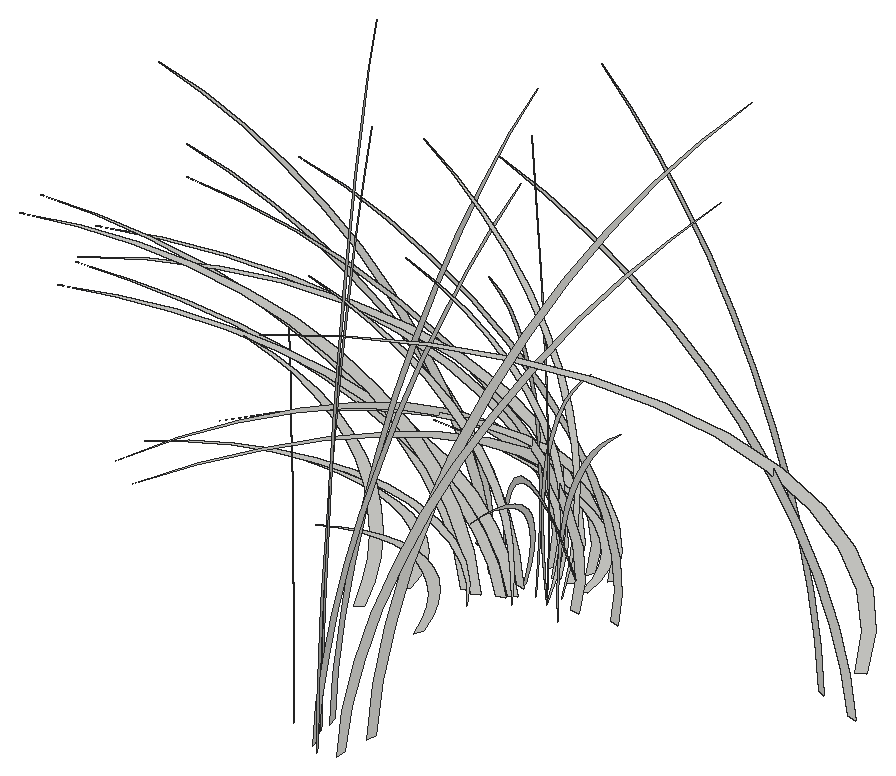
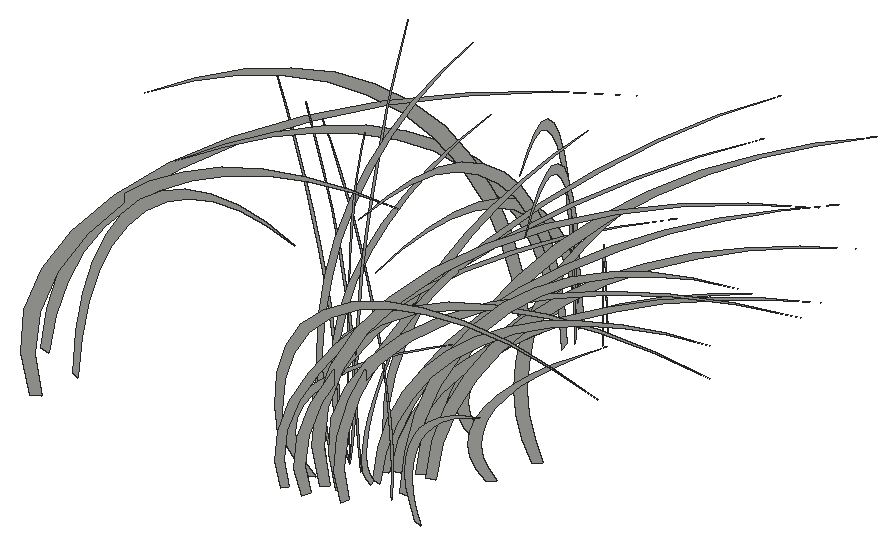
# SketchUp Ruby script. Lengths in inches.
U = 1.inch
M = Sketchup.active_model
def pt(a) = Geom::Point3d.new(a.map { |v| v * U })
def face(e, loops, mat)
  f = e.add_face(loops[0].map { |a| pt(a) })
  loops[1..].each { |l| e.add_face(l.map { |a| pt(a) }).erase! }
  f.material = f.back_material = mat if mat
  f
end
# faces: each face lists its corners as indices into pts; further lists are holes
def faces(e, pts, list, mat = nil) = list.each { |f| face(e, (f[0].is_a?(Array) ? f : [f]).map { |l| l.map { |i| pts[i] } }, mat) }
# xy, xz, yz: faces in a plane at the given z, y or x. An outline is a flat list of corners, or four numbers for a rectangle; further outlines are holes
def ring(l) = l.size == 4 ? [[l[0], l[1]], [l[2], l[1]], [l[2], l[3]], [l[0], l[3]]] : l.each_slice(2).to_a
def flat(e, list, mat, &to3) = list.each { |f| face(e, (f[0].is_a?(Array) ? f : [f]).map { |l| ring(l).map { |u, v| to3.(u, v) } }, mat) }
def xy(e, z, list, mat = nil) = flat(e, list, mat) { |x, y| [x, y, z] }
def xz(e, y, list, mat = nil) = flat(e, list, mat) { |x, z| [x, y, z] }
def yz(e, x, list, mat = nil) = flat(e, list, mat) { |y, z| [x, y, z] }
def lines(e, pts, list) = list.each { |a, b| e.add_line(pt(pts[a]), pt(pts[b])) }
# prism: a flat outline (further loops are holes) pulled along v
def prism(e, loops, v, mat = nil)
  f = face(e, loops, mat); d = Geom::Vector3d.new(v.map { |x| x * U })
  f.pushpull(f.normal.samedirection?(d) ? d.length : -d.length)
end
def box(e, o, s, mat = nil) = prism(e, [[o, [o[0] + s[0], o[1], o[2]], [o[0] + s[0], o[1] + s[1], o[2]], [o[0], o[1] + s[1], o[2]]]], [0, 0, s[2]], mat)
def at(x, y, z, deg = 0) = Geom::Transformation.translation(pt([x, y, z])) * Geom::Transformation.rotation(ORIGIN, Z_AXIS, deg.degrees)
def axes(o, x, y, z) = Geom::Transformation.new([*x, 0, *y, 0, *z, 0, *pt(o).to_a, 1])
def part(name) = M.definitions.add(name)
# library, detail: a bought-in or finely detailed component or shape, given as its bounding box
def library(name, o, s) = part(name).tap { |d| box(d.entities, o, s) }
def detail(e, o, s) = box(e.add_group.entities, o, s)
def put(e, d, t, mat = nil) = e.add_instance(d, t).tap { |i| i.material = mat if mat }
def group(e, t, mat = nil) = e.add_group.tap { |g| g.transformation = t; g.material = mat if mat }.entities
root = M.entities
g1 = group(root,at(15.17,758.32,-58.625))
p = [[-6.5,7.92,6.04],[-5.63,6.85,6],[-4.77,5.81,5.85],[-3.94,4.8,5.6],[-3.16,3.84,5.25],[-2.4375,2.97,4.81],
  [-1.79,2.18,4.28],[-1.23,1.5,3.68],[-0.77,0.9375,3.02],[-0.42,0.51,2.3],[-0.18,0.22,1.55],[-0.06,0.07,0.78],
  [-0.06,0.07,0],[0,0,0.8],[-0.08,0.09,1.59],[-0.28,0.35,2.36],[-0.62,0.76,3.1],[-1.08,1.3125,3.79],
  [-1.64,2,4.41],[-2.31,2.81,4.94],[-3.05,3.72,5.38],[-3.86,4.7,5.72],[-4.72,5.75,5.94],[-5.61,6.83,6.05]]
faces(g1,p,[[0,1,2,3,4,5,6,7,8,9,10,11,12,13,14,15,16,17,18,19,20,21,22,23]])
g2 = group(root,at(15.29,769.34,-58.625))
p = [[-0.14,-0.48,0],[-0.0625,-0.21,0],[0,0,1.01],[-0.03,-0.09,2.03],[-0.14,-0.47,3.02],[-0.33,-1.14,3.98],
  [-0.61,-2.08,4.86],[-0.95,-3.26,5.65],[-1.37,-4.67,6.34],[-1.83,-6.26,6.89],[-2.34,-7.99,7.31],[-2.87,-9.82,7.58],
  [-3.42,-11.7,7.68],[-3.98,-13.6,7.63],[-3.43,-11.74,7.64],[-2.89,-9.9,7.5],[-2.375,-8.12,7.21],[-1.88,-6.44,6.78],
  [-1.43,-4.91,6.22],[-1.04,-3.55,5.54],[-0.7,-2.39,4.76],[-0.43,-1.48,3.89],[-0.24,-0.8125,2.96],[-0.125,-0.42,1.99],
  [-0.09,-0.31,0.99]]
faces(g2,p,[[0,1,2,3,4,5,6,7,8,9,10,11,12,13,14,15,16,17,18,19,20,21,22,23,24]])
g3 = group(root,at(16.34,769.67,-58.625))
p = [[-0.18,-0.47,0],[-0.08,-0.21,0],[0,0,0.88],[-0.03,-0.08,1.76],[-0.17,-0.46,2.63],[-0.42,-1.11,3.46],
  [-0.77,-2.02,4.23],[-1.2,-3.18,4.92],[-1.72,-4.55,5.51],[-2.3,-6.1,6],[-2.94,-7.78,6.36],[-3.62,-9.57,6.59],
  [-4.31,-11.41,6.6875],[-5.01,-13.25,6.64],[-4.32,-11.44,6.65],[-3.65,-9.65,6.53],[-2.99,-7.91,6.28],[-2.37,-6.28,5.9],
  [-1.81,-4.78,5.41],[-1.31,-3.46,4.82],[-0.88,-2.33,4.14],[-0.54,-1.4375,3.39],[-0.3,-0.79,2.58],[-0.16,-0.41,1.73],
  [-0.11,-0.3,0.86]]
faces(g3,p,[[0,1,2,3,4,5,6,7,8,9,10,11,12,13,14,15,16,17,18,19,20,21,22,23,24]])
g4 = group(root,at(14.92,764.6875,-58.625))
p = [[-1.5,-3.28,3.96],[-1.23,-2.68,3.71],[-0.98,-2.14,3.43],[-0.76,-1.66,3.13],[-0.57,-1.25,2.82],[-0.42,-0.91,2.49],
  [-0.29,-0.64,2.15],[-0.21,-0.45,1.79],[-0.16,-0.34,1.43],[-0.14,-0.31,1.07],[-0.16,-0.35,0.71],[-0.22,-0.48,0.35],
  [-0.3125,-0.6875,0],[-0.19,-0.42,0],[-0.09,-0.19,0.36],[-0.02,-0.05,0.72],[0,0,1.09],[-0.02,-0.04,1.46],
  [-0.07,-0.16,1.82],[-0.17,-0.37,2.18],[-0.31,-0.67,2.53],[-0.48,-1.05,2.86],[-0.6875,-1.5,3.17],[-0.93,-2.03,3.46],
  [-1.2,-2.62,3.72]]
faces(g4,p,[[0,1,2,3,4,5,6,7,8,9,10,11,12,13,14,15,16,17,18,19,20,21,22,23,24]])
g5 = group(root,at(14.8,766.07,-58.625))
p = [[-6.52,-5.35,4.97],[-5.64,-4.63,4.9375],[-4.78,-3.92,4.82],[-3.95,-3.24,4.61],[-3.16,-2.6,4.32],[-2.44,-2,3.96],
  [-1.79,-1.47,3.52],[-1.23,-1.01,3.03],[-0.77,-0.64,2.48],[-0.42,-0.34,1.9],[-0.18,-0.15,1.28],[-0.06,-0.05,0.64],
  [-0.06,-0.05,0],[0,0,0.65],[-0.08,-0.0625,1.31],[-0.29,-0.23,1.95],[-0.62,-0.51,2.55],[-1.08,-0.89,3.12],
  [-1.65,-1.35,3.625],[-2.3125,-1.9,4.07],[-3.06,-2.51,4.43],[-3.87,-3.18,4.7],[-4.73,-3.89,4.89],[-5.62,-4.62,4.98]]
faces(g5,p,[[0,1,2,3,4,5,6,7,8,9,10,11,12,13,14,15,16,17,18,19,20,21,22,23]])
g6 = group(root,at(14.67,766.7,-58.625))
p = [[-8.75,-5.68,10.42],[-10.07,-6.54,10.69],[-8.79,-5.71,10.36],[-7.56,-4.91,9.9],[-6.38,-4.14,9.32],[-5.27,-3.42,8.62],
  [-4.25,-2.76,7.81],[-3.32,-2.16,6.9],[-2.5,-1.62,5.9],[-1.79,-1.16,4.83],[-1.2,-0.78,3.6875],[-0.74,-0.48,2.49],
  [-0.42,-0.27,1.26],[-0.23,-0.15,0],[0,0,0],[-0.15,-0.1,1.29],[-0.46,-0.3,2.55],[-0.91,-0.59,3.78],
  [-1.5,-0.97,4.95],[-2.23,-1.45,6.04],[-3.07,-2,7.05],[-4.03,-2.62,7.96],[-5.1,-3.31,8.76],[-6.25,-4.06,9.45],
  [-7.47,-4.85,10]]
faces(g6,p,[[0,1,2,3,4,5,6,7,8,9,10,11,12,13,14,15,16,17,18,19,20,21,22,23,24]])
g7 = group(root,at(13.05,764.64,-58.625))
p = [[-2.79,-2.29,8.05],[-2.28,-1.87,7.53],[-1.82,-1.49,6.97],[-1.41,-1.16,6.37],[-1.06,-0.87,5.73],[-0.77,-0.63,5.06],
  [-0.54,-0.45,4.36],[-0.38,-0.32,3.64],[-0.29,-0.24,2.91],[-0.26,-0.21,2.18],[-0.3,-0.25,1.44],[-0.41,-0.34,0.71],
  [-0.58,-0.48,0],[-0.36,-0.29,0],[-0.16,-0.14,0.72],[-0.04,-0.04,1.46],[0,0,2.21],[-0.03,-0.03,2.96],
  [-0.14,-0.11,3.71],[-0.32,-0.26,4.43],[-0.57,-0.47,5.14],[-0.89,-0.73,5.81],[-1.28,-1.05,6.44],[-1.72,-1.42,7.03],
  [-2.23,-1.83,7.57]]
faces(g7,p,[[0,1,2,3,4,5,6,7,8,9,10,11,12,13,14,15,16,17,18,19,20,21,22,23,24]])
g8 = group(root,at(13.05,764.64,-58.625))
p = [[-2.79,-2.29,8.05],[-2.28,-1.87,7.53],[-1.82,-1.49,6.97],[-1.41,-1.16,6.37],[-1.06,-0.87,5.73],[-0.77,-0.63,5.06],
  [-0.54,-0.45,4.36],[-0.38,-0.32,3.64],[-0.29,-0.24,2.91],[-0.26,-0.21,2.18],[-0.3,-0.25,1.44],[-0.41,-0.34,0.71],
  [-0.58,-0.48,0],[-0.36,-0.29,0],[-0.16,-0.14,0.72],[-0.04,-0.04,1.46],[0,0,2.21],[-0.03,-0.03,2.96],
  [-0.14,-0.11,3.71],[-0.32,-0.26,4.43],[-0.57,-0.47,5.14],[-0.89,-0.73,5.81],[-1.28,-1.05,6.44],[-1.72,-1.42,7.03],
  [-2.23,-1.83,7.57]]
faces(g8,p,[[0,1,2,3,4,5,6,7,8,9,10,11,12,13,14,15,16,17,18,19,20,21,22,23,24]])
g9 = group(root,at(16.57,757.49,-58.625))
p = [[-6.9,10.63,10.21],[-7.94,12.23,10.48],[-6.9375,10.68,10.15],[-5.96,9.18,9.7],[-5.03,7.75,9.13],[-4.16,6.41,8.44],
  [-3.35,5.16,7.65],[-2.62,4.03,6.76],[-1.97,3.03,5.78],[-1.41,2.17,4.73],[-0.95,1.46,3.61],[-0.58,0.9,2.44],
  [-0.33,0.5,1.23],[-0.18,0.28,0],[0,0,0],[-0.12,0.1875,1.26],[-0.36,0.56,2.5],[-0.72,1.1,3.7],
  [-1.18,1.82,4.85],[-1.76,2.7,5.92],[-2.43,3.73,6.91],[-3.18,4.9,7.8],[-4.02,6.19,8.59],[-4.93,7.59,9.26],
  [-5.89,9.08,9.8]]
faces(g9,p,[[0,1,2,3,4,5,6,7,8,9,10,11,12,13,14,15,16,17,18,19,20,21,22,23,24]])
g10 = group(root,at(15.48,767.23,-58.625))
p = [[-8.75,-5.68,8.4],[-10.07,-6.54,8.62],[-8.79,-5.71,8.35],[-7.56,-4.91,7.98],[-6.38,-4.14,7.51],[-5.27,-3.42,6.95],
  [-4.25,-2.76,6.3],[-3.32,-2.16,5.5625],[-2.5,-1.62,4.76],[-1.79,-1.16,3.89],[-1.2,-0.78,2.97],[-0.74,-0.48,2.01],
  [-0.42,-0.27,1.02],[-0.23,-0.15,0],[0,0,0],[-0.15,-0.1,1.04],[-0.46,-0.3,2.06],[-0.91,-0.59,3.05],
  [-1.5,-0.97,3.99],[-2.23,-1.45,4.87],[-3.07,-2,5.6875],[-4.03,-2.62,6.42],[-5.1,-3.31,7.07],[-6.25,-4.06,7.62],
  [-7.47,-4.85,8.0625]]
faces(g10,p,[[0,1,2,3,4,5,6,7,8,9,10,11,12,13,14,15,16,17,18,19,20,21,22,23,24]])
g11 = group(root,at(15.93,758.48,-58.625))
p = [[-6.9,10.63,12.66],[-7.94,12.23,12.99],[-6.9375,10.68,12.59],[-5.96,9.18,12.03],[-5.03,7.75,11.32],[-4.16,6.41,10.47],
  [-3.35,5.16,9.49],[-2.62,4.03,8.38],[-1.97,3.03,7.17],[-1.41,2.17,5.87],[-0.95,1.46,4.48],[-0.58,0.9,3.03],
  [-0.33,0.5,1.53],[-0.18,0.28,0],[0,0,0],[-0.12,0.1875,1.57],[-0.36,0.56,3.1],[-0.72,1.1,4.59],
  [-1.18,1.82,6.01],[-1.76,2.7,7.34],[-2.43,3.73,8.57],[-3.18,4.9,9.68],[-4.02,6.19,10.65],[-4.93,7.59,11.48],
  [-5.89,9.08,12.15]]
faces(g11,p,[[0,1,2,3,4,5,6,7,8,9,10,11,12,13,14,15,16,17,18,19,20,21,22,23,24]])
g12 = group(root,at(14.18,768.25,-58.625))
p = [[0.29,-0.25,0],[0.13,-0.11,0],[0,0,0.73],[0.05,-0.05,1.47],[0.28,-0.25,2.2],[0.68,-0.6,2.89],
  [1.24,-1.09,3.53],[1.95,-1.71,4.11],[2.79,-2.45,4.6],[3.74,-3.29,5.01],[4.77,-4.19,5.3125],[5.87,-5.16,5.51],
  [7,-6.15,5.58],[8.13,-7.14,5.55],[7.02,-6.17,5.55],[5.92,-5.2,5.45],[4.85,-4.26,5.24],[3.85,-3.38,4.93],
  [2.93,-2.58,4.52],[2.12,-1.86,4.03],[1.43,-1.26,3.46],[0.88,-0.78,2.83],[0.49,-0.43,2.15],[0.25,-0.22,1.44],
  [0.18,-0.16,0.72]]
faces(g12,p,[[0,1,2,3,4,5,6,7,8,9,10,11,12,13,14,15,16,17,18,19,20,21,22,23,24]])
g13 = group(root,at(14.18,768.25,-58.625))
p = [[0.29,-0.25,0],[0.13,-0.11,0],[0,0,0.73],[0.05,-0.05,1.47],[0.28,-0.25,2.2],[0.68,-0.6,2.89],
  [1.24,-1.09,3.53],[1.95,-1.71,4.11],[2.79,-2.45,4.6],[3.74,-3.29,5.01],[4.77,-4.19,5.3125],[5.87,-5.16,5.51],
  [7,-6.15,5.58],[8.13,-7.14,5.55],[7.02,-6.17,5.55],[5.92,-5.2,5.45],[4.85,-4.26,5.24],[3.85,-3.38,4.93],
  [2.93,-2.58,4.52],[2.12,-1.86,4.03],[1.43,-1.26,3.46],[0.88,-0.78,2.83],[0.49,-0.43,2.15],[0.25,-0.22,1.44],
  [0.18,-0.16,0.72]]
faces(g13,p,[[0,1,2,3,4,5,6,7,8,9,10,11,12,13,14,15,16,17,18,19,20,21,22,23,24]])
g14 = group(root,at(16.26,757.74,-58.625))
p = [[-3.71,12.12,8.88],[-4.26,13.95,9.11],[-3.72,12.18,8.83],[-3.2,10.47,8.4375],[-2.7,8.84,7.94],[-2.23,7.3,7.34],
  [-1.8,5.89,6.66],[-1.41,4.6,5.88],[-1.06,3.46,5.03],[-0.76,2.48,4.12],[-0.51,1.66,3.14],[-0.3125,1.03,2.125],
  [-0.18,0.58,1.07],[-0.1,0.32,0],[0,0,0],[-0.07,0.21,1.1],[-0.19,0.64,2.18],[-0.39,1.26,3.22],
  [-0.64,2.08,4.22],[-0.94,3.08,5.15],[-1.3,4.26,6.01],[-1.71,5.59,6.79],[-2.16,7.0625,7.47],[-2.65,8.65,8.05],
  [-3.16,10.35,8.52]]
faces(g14,p,[[0,1,2,3,4,5,6,7,8,9,10,11,12,13,14,15,16,17,18,19,20,21,22,23,24]])
g15 = group(root,at(14.35,766.6875,-58.625))
p = [[-9.98,-3.05,9.0625],[-11.48,-3.51,9.3],[-10.02,-3.0625,9.01],[-8.61,-2.63,8.61],[-7.27,-2.22,8.1],[-6.01,-1.84,7.5],
  [-4.84,-1.48,6.79],[-3.79,-1.16,6],[-2.85,-0.87,5.14],[-2.04,-0.62,4.2],[-1.37,-0.42,3.21],[-0.84,-0.26,2.17],
  [-0.47,-0.14,1.1],[-0.26,-0.08,0],[0,0,0],[-0.18,-0.05,1.12],[-0.52,-0.16,2.22],[-1.04,-0.32,3.29],
  [-1.71,-0.52,4.3],[-2.54,-0.78,5.26],[-3.5,-1.07,6.13],[-4.6,-1.41,6.93],[-5.8125,-1.78,7.625],[-7.12,-2.18,8.22],
  [-8.52,-2.6,8.7]]
faces(g15,p,[[0,1,2,3,4,5,6,7,8,9,10,11,12,13,14,15,16,17,18,19,20,21,22,23,24]])
g16 = group(root,at(17.09,757.67,-58.625))
p = [[0.99,12.64,10.21],[1.14,14.54,10.48],[1,12.7,10.15],[0.86,10.91,9.7],[0.72,9.21,9.13],[0.6,7.61,8.44],
  [0.48,6.14,7.65],[0.38,4.79,6.76],[0.28,3.61,5.78],[0.2,2.58,4.73],[0.14,1.73,3.61],[0.08,1.07,2.44],
  [0.05,0.6,1.23],[0.03,0.33,0],[0,0,0],[0.02,0.22,1.26],[0.05,0.66,2.5],[0.1,1.3125,3.7],
  [0.17,2.17,4.85],[0.25,3.21,5.92],[0.35,4.4375,6.91],[0.46,5.83,7.8],[0.58,7.36,8.59],[0.71,9.02,9.26],
  [0.85,10.79,9.8]]
faces(g16,p,[[0,1,2,3,4,5,6,7,8,9,10,11,12,13,14,15,16,17,18,19,20,21,22,23,24]])
g17 = group(root,at(13.37,766.15,-58.625))
p = [[-2.79,-2.29,3.96],[-2.28,-1.87,3.71],[-1.82,-1.49,3.43],[-1.41,-1.16,3.13],[-1.06,-0.87,2.82],[-0.77,-0.63,2.49],
  [-0.54,-0.45,2.15],[-0.38,-0.32,1.79],[-0.29,-0.24,1.43],[-0.26,-0.21,1.07],[-0.3,-0.25,0.71],[-0.41,-0.34,0.35],
  [-0.58,-0.48,0],[-0.36,-0.29,0],[-0.16,-0.14,0.36],[-0.04,-0.04,0.72],[0,0,1.09],[-0.03,-0.03,1.46],
  [-0.14,-0.11,1.82],[-0.32,-0.26,2.18],[-0.57,-0.47,2.53],[-0.89,-0.73,2.86],[-1.28,-1.05,3.17],[-1.72,-1.42,3.46],
  [-2.23,-1.83,3.72]]
faces(g17,p,[[0,1,2,3,4,5,6,7,8,9,10,11,12,13,14,15,16,17,18,19,20,21,22,23,24]])
g18 = group(root,at(15.69,766.8,-58.625))
p = [[-4.12,-3.38,9.85],[-3.46,-2.84,9.12],[-2.86,-2.35,8.37],[-2.3125,-1.9,7.59],[-1.82,-1.49,6.8],[-1.39,-1.14,5.99],
  [-1.01,-0.83,5.16],[-0.7,-0.57,4.32],[-0.44,-0.36,3.47],[-0.25,-0.21,2.61],[-0.12,-0.1,1.74],[-0.06,-0.05,0.87],
  [-0.05,-0.04,0],[0,0,0.875],[-0.02,-0.02,1.75],[-0.11,-0.09,2.625],[-0.28,-0.23,3.49],[-0.52,-0.43,4.35],
  [-0.83,-0.68,5.2],[-1.21,-1,6.03],[-1.66,-1.37,6.84],[-2.18,-1.79,7.63],[-2.77,-2.27,8.4],[-3.41,-2.8,9.14]]
faces(g18,p,[[0,1,2,3,4,5,6,7,8,9,10,11,12,13,14,15,16,17,18,19,20,21,22,23]])
g19 = group(root,at(15.69,766.8,-58.625))
p = [[-4.12,-3.38,9.85],[-3.46,-2.84,9.12],[-2.86,-2.35,8.37],[-2.3125,-1.9,7.59],[-1.82,-1.49,6.8],[-1.39,-1.14,5.99],
  [-1.01,-0.83,5.16],[-0.7,-0.57,4.32],[-0.44,-0.36,3.47],[-0.25,-0.21,2.61],[-0.12,-0.1,1.74],[-0.06,-0.05,0.87],
  [-0.05,-0.04,0],[0,0,0.875],[-0.02,-0.02,1.75],[-0.11,-0.09,2.625],[-0.28,-0.23,3.49],[-0.52,-0.43,4.35],
  [-0.83,-0.68,5.2],[-1.21,-1,6.03],[-1.66,-1.37,6.84],[-2.18,-1.79,7.63],[-2.77,-2.27,8.4],[-3.41,-2.8,9.14]]
faces(g19,p,[[0,1,2,3,4,5,6,7,8,9,10,11,12,13,14,15,16,17,18,19,20,21,22,23]])
g20 = group(root,at(17.04,769.59,-58.625))
p = [[-0.22,-0.31,0],[-0.1,-0.14,0],[0,0,0.84],[-0.04,-0.06,1.69],[-0.22,-0.3,2.53],[-0.53,-0.74,3.32],
  [-0.96,-1.34,4.06],[-1.52,-2.11,4.72],[-2.17,-3.02,5.29],[-2.9,-4.04,5.76],[-3.71,-5.16,6.11],[-4.56,-6.34,6.33],
  [-5.43,-7.5625,6.42],[-6.31,-8.79,6.375],[-5.45,-7.59,6.38],[-4.6,-6.4,6.27],[-3.77,-5.25,6.02],[-2.99,-4.16,5.67],
  [-2.28,-3.17,5.2],[-1.65,-2.29,4.63],[-1.11,-1.55,3.98],[-0.6875,-0.95,3.25],[-0.38,-0.53,2.47],[-0.2,-0.27,1.66],
  [-0.14,-0.2,0.83]]
faces(g20,p,[[0,1,2,3,4,5,6,7,8,9,10,11,12,13,14,15,16,17,18,19,20,21,22,23,24]])
g21 = group(root,at(15.28,766.97,-58.625))
p = [[-9.98,-3.05,7.31],[-11.48,-3.51,7.5],[-10.02,-3.0625,7.27],[-8.61,-2.63,6.94],[-7.27,-2.22,6.54],[-6.01,-1.84,6.04],
  [-4.84,-1.48,5.48],[-3.79,-1.16,4.84],[-2.85,-0.87,4.14],[-2.04,-0.62,3.39],[-1.37,-0.42,2.59],[-0.84,-0.26,1.75],
  [-0.47,-0.14,0.88],[-0.26,-0.08,0],[0,0,0],[-0.18,-0.05,0.9],[-0.52,-0.16,1.79],[-1.04,-0.32,2.65],
  [-1.71,-0.52,3.47],[-2.54,-0.78,4.24],[-3.5,-1.07,4.95],[-4.6,-1.41,5.59],[-5.8125,-1.78,6.15],[-7.12,-2.18,6.63],
  [-8.52,-2.6,7.02]]
faces(g21,p,[[0,1,2,3,4,5,6,7,8,9,10,11,12,13,14,15,16,17,18,19,20,21,22,23,24]])
g22 = group(root,at(25.3,769.83,-58.625))
p = [[-0.46,-0.32,0],[-0.21,-0.14,0],[0,0,1.26],[-0.08,-0.06,2.52],[-0.45,-0.32,3.76],[-1.1,-0.77,4.94],
  [-2.01,-1.4,6.04],[-3.16,-2.2,7.03],[-4.51,-3.15,7.88],[-6.05,-4.22,8.57],[-7.72,-5.39,9.09],[-9.49,-6.625,9.42],
  [-11.32,-7.9,9.56],[-13.15,-9.17,9.49],[-11.35,-7.92,9.51],[-9.57,-6.68,9.33],[-7.85,-5.48,8.97],[-6.23,-4.35,8.44],
  [-4.75,-3.31,7.74],[-3.43,-2.39,6.89],[-2.32,-1.62,5.92],[-1.43,-1,4.84],[-0.79,-0.55,3.68],[-0.41,-0.28,2.47],
  [-0.3,-0.21,1.23]]
faces(g22,p,[[0,1,2,3,4,5,6,7,8,9,10,11,12,13,14,15,16,17,18,19,20,21,22,23,24]])
g23 = group(root,at(16.39,768.85,-58.625))
p = [[-0.39,-0.25,0],[-0.17,-0.11,0],[0,0,1.1875],[-0.07,-0.05,2.38],[-0.38,-0.25,3.56],[-0.93,-0.6,4.68],
  [-1.69,-1.1,5.72],[-2.66,-1.73,6.65],[-3.8,-2.47,7.45],[-5.09,-3.31,8.11],[-6.5,-4.22,8.6],[-7.99,-5.1875,8.91],
  [-9.53,-6.1875,9.04],[-11.07,-7.1875,8.98],[-9.55,-6.2,8.99],[-8.06,-5.23,8.83],[-6.61,-4.29,8.49],[-5.24,-3.41,7.98],
  [-3.99,-2.59,7.32],[-2.89,-1.875,6.52],[-1.95,-1.27,5.6],[-1.2,-0.78,4.58],[-0.66,-0.43,3.48],[-0.34,-0.22,2.34],
  [-0.25,-0.16,1.17]]
faces(g23,p,[[0,1,2,3,4,5,6,7,8,9,10,11,12,13,14,15,16,17,18,19,20,21,22,23,24]])
g24 = group(root,at(17.07,766.87,-58.625))
p = [[4.46,-2.93,8.37],[3.74,-2.46,7.75],[3.09,-2.03,7.11],[2.5,-1.64,6.45],[1.97,-1.29,5.78],[1.5,-0.98,5.09],
  [1.09,-0.72,4.39],[0.75,-0.49,3.67],[0.48,-0.31,2.95],[0.27,-0.18,2.22],[0.13,-0.09,1.48],[0.0625,-0.04,0.74],
  [0.06,-0.04,0],[0,0,0.74],[0.02,-0.01,1.49],[0.12,-0.08,2.23],[0.3,-0.2,2.97],[0.5625,-0.37,3.7],
  [0.9,-0.59,4.42],[1.3125,-0.86,5.13],[1.8,-1.18,5.82],[2.36,-1.55,6.49],[2.99,-1.97,7.14],[3.69,-2.43,7.77]]
faces(g24,p,[[0,1,2,3,4,5,6,7,8,9,10,11,12,13,14,15,16,17,18,19,20,21,22,23]])
g25 = group(root,at(15.91,758.87,-58.625))
p = [[-3.71,12.12,11.01],[-4.26,13.95,11.3],[-3.72,12.18,10.95],[-3.2,10.47,10.46],[-2.7,8.84,9.85],[-2.23,7.3,9.11],
  [-1.8,5.89,8.25],[-1.41,4.6,7.29],[-1.06,3.46,6.24],[-0.76,2.48,5.1],[-0.51,1.66,3.9],[-0.3125,1.03,2.64],
  [-0.18,0.58,1.33],[-0.1,0.32,0],[0,0,0],[-0.07,0.21,1.36],[-0.19,0.64,2.7],[-0.39,1.26,3.99],
  [-0.64,2.08,5.23],[-0.94,3.08,6.39],[-1.3,4.26,7.45],[-1.71,5.59,8.42],[-2.16,7.0625,9.27],[-2.65,8.65,9.99],
  [-3.16,10.35,10.57]]
faces(g25,p,[[0,1,2,3,4,5,6,7,8,9,10,11,12,13,14,15,16,17,18,19,20,21,22,23,24]])
g26 = group(root,at(15.7,767.93,-58.625))
p = [[0.16,-0.45,0],[0.07,-0.2,0.99],[0.02,-0.05,1.99],[0,0,2.99],[0.02,-0.05,3.99],[0.07,-0.2,4.99],
  [0.16,-0.44,5.98],[0.28,-0.79,6.95],[0.4375,-1.23,7.91],[0.625,-1.77,8.85],[0.85,-2.39,9.76],[1.1,-3.11,10.64],
  [1.38,-3.91,11.49],[1.12,-3.16,10.63],[0.88,-2.48,9.74],[0.67,-1.89,8.82],[0.49,-1.375,7.89],[0.34,-0.95,6.93],
  [0.22,-0.61,5.96],[0.13,-0.36,4.97],[0.07,-0.2,3.98],[0.04,-0.125,2.98],[0.05,-0.14,1.98],[0.09,-0.25,0.99]]
faces(g26,p,[[0,1,2,3,4,5,6,7,8,9,10,11,12,13,14,15,16,17,18,19,20,21,22,23]])
g27 = group(root,at(17.18,758.84,-58.625))
p = [[0.99,12.64,12.66],[1.14,14.54,12.99],[1,12.7,12.59],[0.86,10.91,12.03],[0.72,9.21,11.32],[0.6,7.61,10.47],
  [0.48,6.14,9.49],[0.38,4.79,8.38],[0.28,3.61,7.17],[0.2,2.58,5.87],[0.14,1.73,4.48],[0.08,1.07,3.03],
  [0.05,0.6,1.53],[0.03,0.33,0],[0,0,0],[0.02,0.22,1.57],[0.05,0.66,3.1],[0.1,1.3125,4.59],
  [0.17,2.17,6.01],[0.25,3.21,7.34],[0.35,4.4375,8.57],[0.46,5.83,9.68],[0.58,7.36,10.65],[0.71,9.02,11.48],
  [0.85,10.79,12.15]]
faces(g27,p,[[0,1,2,3,4,5,6,7,8,9,10,11,12,13,14,15,16,17,18,19,20,21,22,23,24]])
g28 = group(root,at(15.02,768.48,-58.625))
p = [[1.5,-4.52,3.96],[1.21,-3.66,3.71],[0.95,-2.89,3.43],[0.73,-2.2,3.13],[0.53,-1.61,2.82],[0.37,-1.12,2.49],
  [0.24,-0.74,2.15],[0.15,-0.46,1.79],[0.1,-0.3,1.43],[0.09,-0.26,1.07],[0.11,-0.33,0.71],[0.17,-0.51,0.35],
  [0.26,-0.8,0],[0.2,-0.61,0],[0.09,-0.27,0.35],[0.02,-0.06,0.7],[-0.01,0.03,1.07],[0,-0.01,1.43],
  [0.06,-0.17,1.8],[0.15,-0.46,2.15],[0.29,-0.87,2.5],[0.46,-1.4,2.83],[0.67,-2.03,3.15],[0.92,-2.77,3.44],
  [1.19,-3.6,3.71]]
faces(g28,p,[[0,1,2,3,4,5,6,7,8,9,10,11,12,13,14,15,16,17,18,19,20,21,22,23,24]])
g29 = group(root,at(16.72,767.65,-58.625))
p = [[-0.37,-0.3,0],[-0.16,-0.13,0.89],[-0.04,-0.03,1.79],[0,0,2.69],[-0.04,-0.03,3.6],[-0.16,-0.13,4.49],
  [-0.36,-0.3,5.39],[-0.65,-0.53,6.27],[-1.01,-0.83,7.13],[-1.45,-1.1875,7.97],[-1.96,-1.61,8.79],[-2.55,-2.09,9.59],
  [-3.21,-2.63,10.35],[-2.59,-2.125,9.58],[-2.03,-1.67,8.77],[-1.55,-1.27,7.95],[-1.13,-0.93,7.1],[-0.78,-0.64,6.24],
  [-0.5,-0.41,5.37],[-0.3,-0.24,4.48],[-0.16,-0.13,3.59],[-0.1,-0.09,2.6875],[-0.12,-0.1,1.79],[-0.21,-0.17,0.89]]
faces(g29,p,[[0,1,2,3,4,5,6,7,8,9,10,11,12,13,14,15,16,17,18,19,20,21,22,23]])
g30 = group(root,at(15.95,767.61,-58.625))
p = [[0.4,-0.26,0],[0.18,-0.12,0.76],[0.04,-0.03,1.52],[0,0,2.29],[0.04,-0.03,3.06],[0.18,-0.12,3.82],
  [0.39,-0.26,4.58],[0.7,-0.46,5.33],[1.09,-0.72,6.06],[1.57,-1.03,6.78],[2.12,-1.39,7.48],[2.76,-1.8125,8.15],
  [3.47,-2.28,8.8],[2.8,-1.84,8.14],[2.2,-1.45,7.46],[1.67,-1.1,6.76],[1.22,-0.8,6.04],[0.84,-0.55,5.31],
  [0.54,-0.36,4.5625],[0.32,-0.21,3.81],[0.18,-0.12,3.05],[0.11,-0.07,2.28],[0.13,-0.08,1.52],[0.22,-0.15,0.76]]
faces(g30,p,[[0,1,2,3,4,5,6,7,8,9,10,11,12,13,14,15,16,17,18,19,20,21,22,23]])
g31 = group(root,at(15.97,768.7,-58.625))
p = [[-0.44,-0.14,0],[-0.2,-0.06,0],[0,0,1.03],[-0.08,-0.02,2.07],[-0.43,-0.13,3.09],[-1.06,-0.32,4.07],
  [-1.93,-0.59,4.97],[-3.03,-0.93,5.79],[-4.33,-1.32,6.49],[-5.81,-1.77,7.06],[-7.41,-2.27,7.48],[-9.11,-2.79,7.75],
  [-10.86,-3.32,7.87],[-12.62,-3.86,7.8125],[-10.89,-3.33,7.82],[-9.1875,-2.81,7.68],[-7.54,-2.3,7.38],[-5.98,-1.83,6.94],
  [-4.55,-1.39,6.37],[-3.29,-1.01,5.67],[-2.22,-0.68,4.87],[-1.37,-0.42,3.98],[-0.75,-0.23,3.03],[-0.39,-0.12,2.03],
  [-0.29,-0.09,1.02]]
faces(g31,p,[[0,1,2,3,4,5,6,7,8,9,10,11,12,13,14,15,16,17,18,19,20,21,22,23,24]])
g32 = group(root,at(16.87,768.05,-58.625))
p = [[-0.43,-0.2,0],[-0.19,-0.09,1.14],[-0.05,-0.02,2.28],[0,0,3.4375],[-0.05,-0.02,4.59],[-0.19,-0.09,5.73],
  [-0.43,-0.2,6.87],[-0.76,-0.36,7.99],[-1.18,-0.55,9.1],[-1.7,-0.79,10.17],[-2.3,-1.08,11.22],[-2.99,-1.4,12.23],
  [-3.76,-1.76,13.21],[-3.03,-1.42,12.22],[-2.38,-1.12,11.2],[-1.8125,-0.85,10.14],[-1.32,-0.62,9.0625],[-0.91,-0.43,7.96],
  [-0.59,-0.27,6.85],[-0.35,-0.16,5.71],[-0.19,-0.09,4.57],[-0.12,-0.06,3.43],[-0.14,-0.06,2.28],[-0.24,-0.11,1.14]]
faces(g32,p,[[0,1,2,3,4,5,6,7,8,9,10,11,12,13,14,15,16,17,18,19,20,21,22,23]])
g33 = group(root,at(17.35,768.78,-58.625))
p = [[-4.36,-1.93,4.55],[-3.53,-1.5625,4.26],[-2.78,-1.23,3.94],[-2.12,-0.9375,3.6],[-1.55,-0.6875,3.24],[-1.08,-0.48,2.86],
  [-0.71,-0.3125,2.47],[-0.45,-0.2,2.06],[-0.29,-0.13,1.65],[-0.25,-0.11,1.23],[-0.3125,-0.14,0.82],[-0.49,-0.22,0.4],
  [-0.77,-0.34,0],[-0.58,-0.26,0],[-0.26,-0.12,0.4],[-0.06,-0.02,0.81],[0.03,0.01,1.23],[-0.01,0,1.65],
  [-0.17,-0.07,2.06],[-0.44,-0.2,2.47],[-0.84,-0.37,2.875],[-1.34,-0.6,3.26],[-1.96,-0.87,3.62],[-2.67,-1.18,3.96],
  [-3.47,-1.54,4.27]]
faces(g33,p,[[0,1,2,3,4,5,6,7,8,9,10,11,12,13,14,15,16,17,18,19,20,21,22,23,24]])
g34 = group(root,at(17.49,767.49,-58.625))
p = [[-0.5,0.04,0],[-0.22,0.02,0],[0,0,1.01],[-0.09,0.01,2.03],[-0.49,0.04,3.02],[-1.18,0.09,3.98],
  [-2.16,0.17,4.86],[-3.39,0.27,5.65],[-4.85,0.38,6.34],[-6.5,0.51,6.89],[-8.29,0.65,7.31],[-10.2,0.8,7.58],
  [-12.16,0.96,7.68],[-14.125,1.11,7.63],[-12.19,0.96,7.64],[-10.28,0.81,7.5],[-8.43,0.66,7.21],[-6.69,0.53,6.78],
  [-5.1,0.4,6.22],[-3.68,0.29,5.54],[-2.49,0.2,4.76],[-1.53,0.12,3.89],[-0.84,0.07,2.96],[-0.4375,0.03,1.99],
  [-0.32,0.03,0.99]]
faces(g34,p,[[0,1,2,3,4,5,6,7,8,9,10,11,12,13,14,15,16,17,18,19,20,21,22,23,24]])
g35 = group(root,at(15.34,767.66,-58.625))
p = [[-10.4,0.82,8.4],[-11.97,0.94,8.62],[-10.45,0.82,8.35],[-8.98,0.71,7.98],[-7.58,0.6,7.51],[-6.27,0.49,6.95],
  [-5.05,0.4,6.3],[-3.95,0.3125,5.5625],[-2.97,0.23,4.76],[-2.125,0.17,3.89],[-1.43,0.11,2.97],[-0.88,0.07,2.01],
  [-0.49,0.04,1.02],[-0.27,0.02,0],[0,0,0],[-0.18,0.01,1.04],[-0.54,0.04,2.06],[-1.08,0.09,3.05],
  [-1.78,0.14,3.99],[-2.64,0.21,4.87],[-3.65,0.29,5.6875],[-4.8,0.38,6.42],[-6.06,0.48,7.07],[-7.43,0.58,7.62],
  [-8.88,0.7,8.0625]]
faces(g35,p,[[0,1,2,3,4,5,6,7,8,9,10,11,12,13,14,15,16,17,18,19,20,21,22,23,24]])
g36 = group(root,at(14.37,767.73,-58.625))
p = [[-10.4,0.82,10.42],[-11.97,0.94,10.69],[-10.45,0.82,10.36],[-8.98,0.71,9.9],[-7.58,0.6,9.32],[-6.27,0.49,8.62],
  [-5.05,0.4,7.81],[-3.95,0.3125,6.9],[-2.97,0.23,5.9],[-2.125,0.17,4.83],[-1.43,0.11,3.6875],[-0.88,0.07,2.49],
  [-0.49,0.04,1.26],[-0.27,0.02,0],[0,0,0],[-0.18,0.01,1.29],[-0.54,0.04,2.55],[-1.08,0.09,3.78],
  [-1.78,0.14,4.95],[-2.64,0.21,6.04],[-3.65,0.29,7.05],[-4.8,0.38,7.96],[-6.06,0.48,8.76],[-7.43,0.58,9.45],
  [-8.88,0.7,10]]
faces(g36,p,[[0,1,2,3,4,5,6,7,8,9,10,11,12,13,14,15,16,17,18,19,20,21,22,23,24]])
g37 = group(root,at(16.6875,767.01,-58.625))
p = [[-0.34,0.34,0],[-0.15,0.15,1.02],[-0.04,0.04,2.06],[0,0,3.1],[-0.04,0.04,4.13],[-0.15,0.15,5.17],
  [-0.33,0.33,6.19],[-0.59,0.59,7.2],[-0.92,0.92,8.19],[-1.32,1.32,9.16],[-1.8,1.8,10.11],[-2.33,2.33,11.02],
  [-2.93,2.93,11.9],[-2.37,2.37,11.01],[-1.86,1.86,10.09],[-1.41,1.41,9.14],[-1.03,1.03,8.17],[-0.71,0.71,7.17],
  [-0.46,0.46,6.17],[-0.27,0.27,5.15],[-0.15,0.15,4.12],[-0.09,0.09,3.09],[-0.11,0.11,2.06],[-0.1875,0.1875,1.02]]
faces(g37,p,[[0,1,2,3,4,5,6,7,8,9,10,11,12,13,14,15,16,17,18,19,20,21,22,23]])
g38 = group(root,at(26.42,767.56,-58.625))
p = [[-12.4,2.64,10.21],[-14.27,3.03,10.48],[-12.46,2.65,10.15],[-10.71,2.28,9.7],[-9.04,1.92,9.13],[-7.47,1.59,8.44],
  [-6.02,1.28,7.65],[-4.7,1,6.76],[-3.54,0.75,5.78],[-2.53,0.54,4.73],[-1.7,0.36,3.61],[-1.05,0.22,2.44],
  [-0.59,0.125,1.23],[-0.32,0.07,0],[0,0,0],[-0.22,0.05,1.26],[-0.65,0.14,2.5],[-1.29,0.27,3.7],
  [-2.125,0.45,4.85],[-3.15,0.67,5.92],[-4.36,0.93,6.91],[-5.72,1.22,7.8],[-7.22,1.54,8.59],[-8.85,1.88,9.26],
  [-10.58,2.25,9.8]]
faces(g38,p,[[0,1,2,3,4,5,6,7,8,9,10,11,12,13,14,15,16,17,18,19,20,21,22,23,24]])
g39 = group(root,at(13.57,768.51,-58.625))
p = [[-3.41,1.17,4.55],[-2.78,0.96,4.26],[-2.22,0.77,3.94],[-1.72,0.59,3.6],[-1.3,0.45,3.24],[-0.94,0.32,2.86],
  [-0.67,0.23,2.47],[-0.47,0.16,2.06],[-0.35,0.12,1.65],[-0.32,0.11,1.23],[-0.37,0.13,0.82],[-0.5,0.17,0.4],
  [-0.71,0.25,0],[-0.4375,0.15,0],[-0.2,0.07,0.41],[-0.05,0.02,0.83],[0,0,1.25],[-0.04,0.01,1.68],
  [-0.17,0.06,2.1],[-0.39,0.13,2.51],[-0.69,0.24,2.9],[-1.09,0.375,3.28],[-1.5625,0.54,3.64],[-2.11,0.73,3.98],
  [-2.73,0.9375,4.28]]
faces(g39,p,[[0,1,2,3,4,5,6,7,8,9,10,11,12,13,14,15,16,17,18,19,20,21,22,23,24]])
g40 = group(root,at(18.66,767.58,-58.625))
p = [[-0.48,0.13,0],[-0.21,0.06,0],[0,0,1.01],[-0.09,0.02,2.03],[-0.47,0.13,3.02],[-1.14,0.31,3.98],
  [-2.09,0.5625,4.86],[-3.28,0.89,5.65],[-4.7,1.27,6.34],[-6.29,1.7,6.89],[-8.03,2.17,7.31],[-9.875,2.66,7.58],
  [-11.77,3.18,7.68],[-13.68,3.69,7.63],[-11.81,3.1875,7.64],[-9.96,2.6875,7.5],[-8.17,2.2,7.21],[-6.48,1.75,6.78],
  [-4.94,1.33,6.22],[-3.57,0.96,5.54],[-2.41,0.65,4.76],[-1.48,0.4,3.89],[-0.82,0.22,2.96],[-0.42,0.11,1.99],
  [-0.3125,0.08,0.99]]
faces(g40,p,[[0,1,2,3,4,5,6,7,8,9,10,11,12,13,14,15,16,17,18,19,20,21,22,23,24]])
g41 = group(root,at(24.98,768.0625,-58.625))
p = [[-11.19,5.95,11.01],[-12.88,6.85,11.3],[-11.24,5.98,10.95],[-9.66,5.14,10.46],[-8.16,4.34,9.85],[-6.74,3.59,9.11],
  [-5.43,2.89,8.25],[-4.25,2.26,7.29],[-3.19,1.7,6.24],[-2.29,1.22,5.1],[-1.53,0.82,3.9],[-0.95,0.5,2.64],
  [-0.53,0.28,1.33],[-0.29,0.16,0],[0,0,0],[-0.2,0.1,1.36],[-0.59,0.3125,2.7],[-1.16,0.62,3.99],
  [-1.92,1.02,5.23],[-2.85,1.51,6.39],[-3.93,2.09,7.45],[-5.16,2.74,8.42],[-6.52,3.47,9.27],[-7.99,4.25,9.99],
  [-9.55,5.08,10.57]]
faces(g41,p,[[0,1,2,3,4,5,6,7,8,9,10,11,12,13,14,15,16,17,18,19,20,21,22,23,24]])
